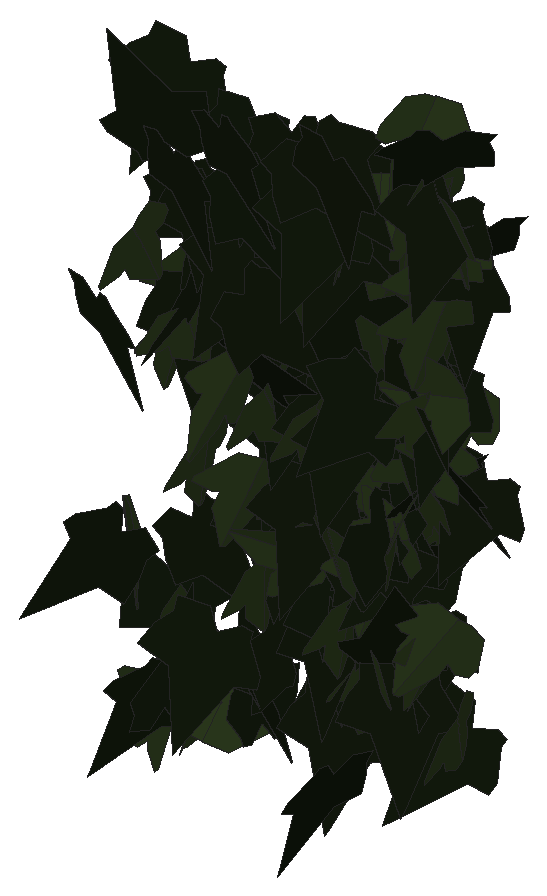
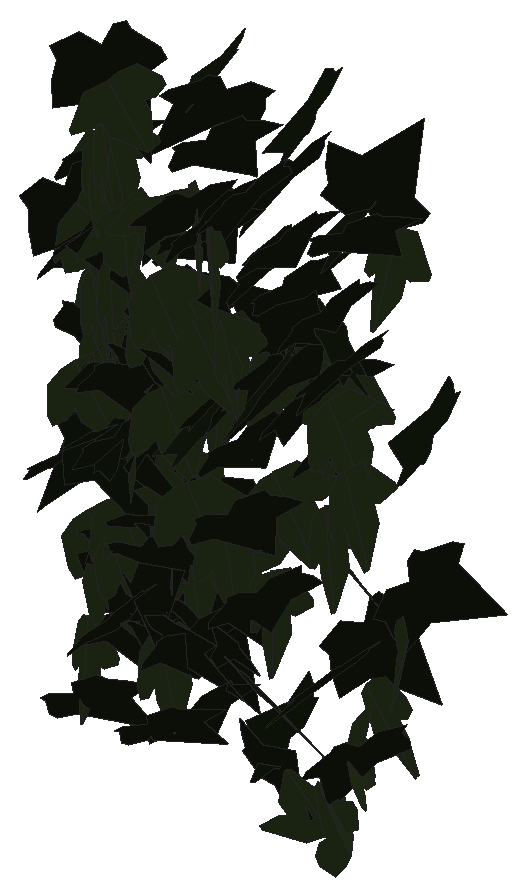
# SketchUp Ruby script. Lengths in inches.
U = 1.inch
M = Sketchup.active_model
def pt(a) = Geom::Point3d.new(a.map { |v| v * U })
def face(e, loops, mat)
  f = e.add_face(loops[0].map { |a| pt(a) })
  loops[1..].each { |l| e.add_face(l.map { |a| pt(a) }).erase! }
  f.material = f.back_material = mat if mat
  f
end
# faces: each face lists its corners as indices into pts; further lists are holes
def faces(e, pts, list, mat = nil) = list.each { |f| face(e, (f[0].is_a?(Array) ? f : [f]).map { |l| l.map { |i| pts[i] } }, mat) }
# xy, xz, yz: faces in a plane at the given z, y or x. An outline is a flat list of corners, or four numbers for a rectangle; further outlines are holes
def ring(l) = l.size == 4 ? [[l[0], l[1]], [l[2], l[1]], [l[2], l[3]], [l[0], l[3]]] : l.each_slice(2).to_a
def flat(e, list, mat, &to3) = list.each { |f| face(e, (f[0].is_a?(Array) ? f : [f]).map { |l| ring(l).map { |u, v| to3.(u, v) } }, mat) }
def xy(e, z, list, mat = nil) = flat(e, list, mat) { |x, y| [x, y, z] }
def xz(e, y, list, mat = nil) = flat(e, list, mat) { |x, z| [x, y, z] }
def yz(e, x, list, mat = nil) = flat(e, list, mat) { |y, z| [x, y, z] }
def lines(e, pts, list) = list.each { |a, b| e.add_line(pt(pts[a]), pt(pts[b])) }
# prism: a flat outline (further loops are holes) pulled along v
def prism(e, loops, v, mat = nil)
  f = face(e, loops, mat); d = Geom::Vector3d.new(v.map { |x| x * U })
  f.pushpull(f.normal.samedirection?(d) ? d.length : -d.length)
end
def box(e, o, s, mat = nil) = prism(e, [[o, [o[0] + s[0], o[1], o[2]], [o[0] + s[0], o[1] + s[1], o[2]], [o[0], o[1] + s[1], o[2]]]], [0, 0, s[2]], mat)
def at(x, y, z, deg = 0) = Geom::Transformation.translation(pt([x, y, z])) * Geom::Transformation.rotation(ORIGIN, Z_AXIS, deg.degrees)
def axes(o, x, y, z) = Geom::Transformation.new([*x, 0, *y, 0, *z, 0, *pt(o).to_a, 1])
def part(name) = M.definitions.add(name)
# library, detail: a bought-in or finely detailed component or shape, given as its bounding box
def library(name, o, s) = part(name).tap { |d| box(d.entities, o, s) }
def detail(e, o, s) = box(e.add_group.entities, o, s)
def put(e, d, t, mat = nil) = e.add_instance(d, t).tap { |i| i.material = mat if mat }
def group(e, t, mat = nil) = e.add_group.tap { |g| g.transformation = t; g.material = mat if mat }.entities
root = M.entities
M.materials.add("efeu1").color = [18, 25, 13]
M.materials.add("efeu2").color = [43, 57, 29]
c1 = part("ivyleaf_9")
p = [[1.54,2.16,1.25],[1.36,2.04,1.19],[-0.21,0.99,0.68],[-0.71,1.11,0.82],[-0.85,0.86,0.67],[-0.8,0.17,0.21],
  [-0.9,-0.01,0.1],[-0.67,-0.16,-0.02],[-0.08,-0.08,-0.05],[-0.03,-0.6,-0.4],[0.65,-0.88,-0.66],[0.83,-0.6,-0.49],
  [1.29,-0.42,-0.43],[1.8125,-0.07,-0.26],[1.21,0.44,0.15]]
faces(c1.entities,p,[[0,1,2,3,4,5,6,7,8,9,10,11,12,13,14]],"efeu1")
c2 = part("ivyleaf_10")
p = [[0,0.5,-0.03],[-0.0625,2.02,-0.43],[-0.19,2.01,-0.46],[-0.54,1.05,-0.29],[-0.52,0.625,-0.18],[-0.83,0.76,-0.28],
  [-1.16,0.64,-0.33],[-1.15,0.33,-0.24],[-0.77,-0.39,0.02],[-0.3,-0.51,0.16],[0.04,-0.48,0.23],[-0.02,2.01,-0.4375],
  [-0.06,2.01,-0.43],[0.04,-0.49,0.23],[0.67,-0.49,0.14],[1.38,0.36,-0.2],[1.375,0.51,-0.24],[0.81,0.65,-0.19],
  [0.62,0.59,-0.15],[0.6,1.09,-0.28],[0.5,1.23,-0.31]]
faces(c2.entities,p,[[0,1,2,3,4,5,6,7,8,9,10],[11,12,0,13,14,15,16,17,18,19,20]],"efeu2")
put(root,c1,axes([18.32,219.18,236.73],[-0.23264,-0.44225,0.01707],[-0.00023,-0.01917,-0.49963],[0.44258,-0.23247,0.00871]))
put(root,c1,axes([16.73,220.26,234.84],[-0.41806,0.26897,-0.05368],[-0.04503,0.02923,0.49711],[0.27055,0.42048,-0.00022]))
put(root,c1,axes([16.32,220.77,234.73],[-0.03728,0.22663,-0.44413],[0.03796,-0.44279,-0.22913],[-0.49716,-0.0508,0.01581]))
put(root,c1,axes([18.61,220.97,234.19],[-0.14053,0.35347,-0.32451],[0.12423,-0.29981,-0.38037],[-0.46348,-0.18754,-0.00356]))
put(root,c2,axes([16.85,221.3,238.65],[-0.03382,-0.35156,0.35392],[0.07856,-0.35406,-0.3442],[0.49263,0.03233,0.07919]))
put(root,c1,axes([15.15,221.35,235.99],[-0.0489,0.0124,-0.49745],[0.08672,-0.49198,-0.02079],[-0.48999,-0.08831,0.04597]))
put(root,c1,axes([16.74,221.28,241.86],[0.30318,-0.39627,0.03242],[0.01873,-0.02649,-0.49895],[0.39716,0.30375,-0.00122]))
put(root,c2,axes([15.68,221.03,240.26],[-0.05258,-0.42552,-0.25722],[0.05175,0.25257,-0.4284],[0.49453,-0.07167,0.01748]))
put(root,c1,axes([18.18,221.54,241.85],[0.10438,-0.44639,0.1996],[0.08744,-0.18377,-0.45671],[0.4811,0.13025,0.0397]))
put(root,c2,axes([15.81,221.17,234.05],[0.30473,-0.15471,-0.36497],[-0.30444,0.2035,-0.34045],[0.25389,0.42971,0.02982]))
put(root,c1,axes([17.23,221.16,239.92],[0.2378,-0.27578,-0.34263],[-0.1,0.3454,-0.34741],[0.42831,0.23376,0.10912]))
put(root,c1,axes([18.04,221.65,241.18],[-0.25106,-0.43024,0.04313],[-0.01388,-0.04182,-0.49805],[0.43218,-0.25128,0.00905]))
put(root,c1,axes([16.83,221.57,238.78],[0.14685,-0.20573,0.4314],[0.35509,-0.25512,-0.24253],[0.31991,0.37761,0.07118]))
put(root,c1,axes([16.91,221.47,241.18],[0.19496,-0.41259,-0.20435],[-0.04645,0.20315,-0.4545],[0.45808,0.1962,0.04089]))
put(root,c1,axes([18.41,221.92,238.65],[-0.21172,-0.34785,0.29012],[-0.08049,-0.28626,-0.40197],[0.44575,-0.21692,0.06522]))
put(root,c1,axes([15.67,221.77,240.95],[0.22727,-0.42698,0.12662],[0.05743,-0.11287,-0.4837],[0.44164,0.2344,-0.00227]))
put(root,c1,axes([16.61,221.98,239.84],[-0.20246,-0.4206,0.17917],[-0.03577,-0.18077,-0.4648],[0.45577,-0.20103,0.04311]))
put(root,c1,axes([15.53,221.71,241.21],[0.2633,0.00372,0.42504],[-0.40216,0.16407,0.24769],[-0.13763,-0.4723,0.08939]))
put(root,c1,axes([17.86,221.6,241.89],[0.0503,-0.31932,-0.38145],[0.12354,0.3794,-0.30132],[0.48188,-0.06394,0.11707]))
put(root,c1,axes([14.42,221.92,238.53],[0.25872,-0.39136,0.17292],[0.09076,-0.14728,-0.46912],[0.41812,0.27413,-0.00517]))
put(root,c2,axes([18.66,222.17,236.97],[-0.07736,-0.11441,-0.48055],[0.13485,-0.47282,0.09087],[-0.47522,-0.11555,0.10402]))
put(root,c2,axes([17.06,221.7,238.32],[-0.07373,-0.42957,-0.24503],[0.04093,0.24158,-0.43585],[0.49284,-0.08433,-0.00046]))
put(root,c2,axes([16.63,222.03,237.02],[-0.23145,-0.40306,0.18432],[-0.07141,-0.17131,-0.46428],[0.43742,-0.24124,0.02174]))
put(root,c1,axes([15.95,221.99,239.49],[-0.39783,0.22915,-0.19804],[0.15833,-0.12137,-0.45848],[-0.25819,-0.4275,0.024]))
put(root,c1,axes([17.97,222.1,238.28],[-0.28766,-0.39412,-0.10918],[0.05279,0.09658,-0.48774],[0.40554,-0.29214,-0.01395]))
put(root,c2,axes([17.95,221.85,236.67],[-0.46075,0.18587,0.05623],[-0.0491,0.02855,-0.49676],[-0.18788,-0.46329,-0.00806]))
put(root,c2,axes([17.62,221.91,238.19],[-0.08403,-0.47039,-0.14723],[0.02547,0.14501,-0.47783],[0.49223,-0.0878,-0.00041]))
put(root,c2,axes([17.97,222.04,235.68],[-0.00171,-0.49775,-0.04733],[-0.00317,0.04734,-0.49774],[0.49999,-0.0014,-0.00332]))
put(root,c1,axes([17.42,222.25,236.87],[-0.39882,-0.26524,-0.1435],[0.11149,0.09139,-0.47877],[0.2802,-0.41388,-0.01375]))
put(root,c2,axes([17.25,222.3,236.01],[-0.22491,-0.02122,-0.44606],[-0.39098,-0.23194,0.20817],[-0.21575,0.44244,0.08774]))
put(root,c1,axes([18.64,222.28,234.76],[-0.12522,-0.47341,-0.10099],[0.03102,0.09625,-0.48967],[0.48307,-0.1289,0.00527]))
put(root,c2,axes([19.17,222.21,239.9],[-0.19706,-0.44281,0.12282],[-0.03389,-0.11927,-0.48438],[0.45828,-0.19923,0.01699]))
put(root,c1,axes([17.65,222.43,240.4],[-0.19809,-0.45502,0.06099],[-0.01773,-0.05879,-0.49622],[0.45875,-0.19875,0.00715]))
put(root,c2,axes([19.22,222.3125,235.72],[-0.33247,-0.21482,0.30548],[-0.19164,-0.25289,-0.38642],[0.32053,-0.37403,0.08582]))
put(root,c2,axes([15.61,222.07,238.72],[-0.21385,-0.42574,-0.15169],[0.06387,0.13767,-0.47641],[0.44742,-0.22314,-0.00449]))
put(root,c1,axes([18.51,222.28,235.16],[0.42159,0.14651,0.22537],[-0.21114,-0.07897,0.4463],[0.16637,-0.47149,-0.00472]))
put(root,c2,axes([14.61,222.26,235.63],[-0.25247,0.37667,-0.21066],[0.07631,-0.20125,-0.4513],[-0.42478,-0.26003,0.04413]))
put(root,c1,axes([19.25,222.17,242.23],[0.03336,0.39852,-0.30011],[-0.14272,-0.28059,-0.38846],[-0.47804,0.11158,0.09503]))
put(root,c2,axes([16.62,222.18,235.7],[0.00602,-0.4867,-0.11438],[0.02004,0.11453,-0.48629],[0.49956,0.00127,0.02088]))
put(root,c1,axes([16.46,222.17,238.91],[0.11594,-0.38414,-0.29831],[-0.02135,0.30236,-0.39765],[0.4859,0.10495,0.05371]))
put(root,c2,axes([18.53,222.24,236.72],[-0.20701,-0.01525,0.45488],[-0.44379,-0.10411,-0.20545],[0.10098,-0.4888,0.02956]))
put(root,c2,axes([19.3,222.2,238.89],[0.1276,0.00772,-0.48338],[-0.46928,0.12209,-0.12193],[0.11615,0.4848,0.03841]))
put(root,c1,axes([19.04,222.56,241.14],[-0.16248,-0.46749,0.0711],[0.00272,-0.07611,-0.49417],[0.47285,-0.1602,0.02727]))
put(root,c1,axes([18.38,222.02,236.96],[0.17794,-0.18481,-0.42916],[-0.16383,0.4054,-0.24251],[0.4376,0.22692,0.08372]))
put(root,c2,axes([17.79,222.23,240.62],[0.26568,-0.39245,-0.15937],[-0.03363,0.16799,-0.46973],[0.42224,0.26032,0.06287]))
put(root,c2,axes([18.22,222.43,236.27],[-0.28434,-0.38052,0.15607],[-0.01846,-0.17774,-0.46698],[0.41086,-0.27132,0.08703]))
put(root,c1,axes([17.55,222.56,233.95],[-0.11709,-0.48526,0.02853],[0.01396,-0.03269,-0.49874],[0.4859,-0.116,0.0212]))
put(root,c1,axes([15.6,222.55,240.0625],[-0.027,-0.49804,0.035],[-0.00041,-0.03503,-0.49877],[0.49927,-0.02696,0.00148]))
put(root,c1,axes([16.13,222.53,234.0625],[0.2143,-0.37408,0.25325],[0.15282,-0.20374,-0.43027],[0.42511,0.26182,0.02701]))
put(root,c2,axes([15.6875,222.29,236.97],[0.01927,-0.48982,-0.09851],[-0.01226,0.09809,-0.49013],[0.49948,0.0213,-0.00823]))
put(root,c1,axes([18.375,222.16,236.11],[-0.46994,0.0383,0.1664],[0.16591,-0.01279,0.4715],[0.04038,0.49837,-0.00069]))
put(root,c2,axes([18.93,222.3,238.61],[-0.168,-0.4604,-0.09903],[0.02599,0.09592,-0.49002],[0.47021,-0.16979,-0.0083]))
put(root,c1,axes([17.86,222.53,239.47],[0.02695,0.18098,-0.46532],[-0.11466,-0.4513,-0.18217],[-0.48593,0.11652,0.01718]))
put(root,c1,axes([16.79,222.51,241.28],[0.08568,-0.48537,-0.08409],[0.00185,0.08567,-0.4926],[0.4926,0.0841,0.01648]))
put(root,c1,axes([17.38,222.57,235.18],[-0.32045,-0.20771,-0.32275],[0.34459,0.02945,-0.36109],[0.16901,-0.45386,0.12427]))
put(root,c2,axes([18.9,222.57,235.4],[0.02016,-0.46392,0.18539],[-0.0018,-0.18561,-0.46427],[0.49959,0.01805,-0.00916]))
put(root,c2,axes([14.94,222.71,234.29],[0.17434,-0.2912,0.36716],[0.22857,-0.28915,-0.33786],[0.4091,0.28565,0.0323]))
put(root,c1,axes([17.29,222.76,240.8],[-0.05143,-0.47217,0.15625],[-0.02724,-0.15417,-0.47486],[0.4966,-0.05736,-0.00986]))
put(root,c1,axes([15.25,222.66,238.54],[0.00132,-0.49997,-0.00532],[0.00004,0.00532,-0.49997],[0.5,0.00132,0.00006]))
put(root,c1,axes([16.8,222.4,234.52],[-0.38182,0.27662,0.16641],[-0.16391,0.05592,-0.46905],[-0.27811,-0.41274,0.04798]))
put(root,c1,axes([19.02,222.61,238.79],[-0.40371,-0.20599,-0.21116],[0.17929,0.11287,-0.4529],[0.23425,-0.44139,-0.01727]))
put(root,c2,axes([18.41,222.1875,234.71],[-0.1228,0.23164,-0.42575],[-0.21963,0.36493,0.2619],[0.43207,0.25134,0.01212]))
put(root,c1,axes([18.54,222.65,239.01],[0.17897,-0.46572,0.03273],[0.00764,-0.03213,-0.49891],[0.46681,0.17908,-0.00439]))
put(root,c1,axes([15.02,222.8,241.48],[-0.29136,-0.40062,0.06792],[0.01585,-0.09471,-0.49069],[0.40603,-0.28378,0.06789]))
put(root,c1,axes([17.0625,222.49,238.44],[0.15996,-0.4199,-0.21932],[-0.02937,0.22225,-0.44693],[0.47281,0.15586,0.04644]))
put(root,c1,axes([16.66,222.79,238.05],[-0.11535,-0.48244,0.06282],[-0.00827,-0.0626,-0.496],[0.48644,-0.11547,0.00646]))
put(root,c2,axes([18.73,222.45,237.8],[-0.42978,-0.21282,-0.14142],[0.13678,0.04214,-0.47908],[0.21583,-0.45048,0.022]))
put(root,c2,axes([18.22,222.45,239.13],[-0.49878,0.0219,0.0272],[-0.02717,0.00119,-0.49926],[-0.02193,-0.49952,0]))
put(root,c1,axes([16.02,222.83,241.01],[-0.06861,-0.49096,0.0652],[0.01069,-0.06728,-0.49534],[0.49516,-0.06657,0.01973]))
put(root,c2,axes([18.9,222.68,240.15],[-0.25963,-0.40554,0.13465],[-0.02665,-0.14188,-0.47871],[0.42647,-0.25575,0.05206]))
put(root,c1,axes([18.48,222.9375,236.29],[-0.39007,-0.2742,0.15052],[-0.04933,-0.18366,-0.46242],[0.30889,-0.37561,0.11623]))
put(root,c2,axes([18.74,222.47,237.33],[-0.41504,0.14577,0.23768],[-0.22998,0.06199,-0.43962],[-0.15764,-0.47424,0.01559]))
put(root,c2,axes([17.92,222.67,234.65],[-0.05427,-0.49609,0.0309],[-0.00255,-0.03081,-0.49904],[0.49704,-0.05432,0.00081]))
put(root,c2,axes([18.625,222.71,242.1],[0.24829,0.38345,-0.20326],[-0.16623,-0.13229,-0.45262],[-0.4009,0.29234,0.06179]))
put(root,c2,axes([17.4,222.76,236.92],[-0.35589,-0.29795,0.18592],[-0.0752,-0.19391,-0.45469],[0.34306,-0.3516,0.09321]))
put(root,c2,axes([18.71,222.73,241.32],[-0.07956,-0.48753,0.07734],[-0.00182,-0.07805,-0.49387],[0.49363,-0.07886,0.01064]))
put(root,c1,axes([18.23,222.5,236.19],[0.16253,0.43439,-0.18679],[-0.06704,-0.17435,-0.4638],[-0.46807,0.17581,0.00157]))
put(root,c1,axes([18.03,222.9,236.13],[-0.3381,-0.35851,-0.08458],[0.07662,0.04385,-0.49215],[0.3603,-0.34575,0.02528]))
put(root,c2,axes([15.27,222.6,232.95],[0.21321,-0.42925,0.14244],[-0.06441,0.12705,0.47928],[-0.44765,-0.22273,-0.00111]))
put(root,c2,axes([16.91,222.74,236.62],[-0.14033,-0.47918,0.02631],[0.00625,-0.02924,-0.49911],[0.47986,-0.13975,0.01419]))
put(root,c2,axes([19.15,222.55,234.36],[0.05969,-0.4314,-0.24562],[-0.02822,0.24404,-0.43549],[0.49562,0.06585,0.00478]))
put(root,c2,axes([19,222.6,241.03],[-0.40372,0.29431,0.01987],[-0.01497,0.0132,-0.4996],[-0.2946,-0.40399,-0.00185]))
put(root,c1,axes([18.48,222.89,238.49],[-0.16875,-0.46052,-0.0972],[0.04425,0.08728,-0.49033],[0.46858,-0.17409,0.0113]))
put(root,c2,axes([17.74,222.83,238.14],[-0.29924,-0.36542,0.16409],[-0.02938,-0.18424,-0.46389],[0.39949,-0.28727,0.08879]))
put(root,c2,axes([16.86,222.7,239.33],[0.07444,-0.48921,-0.07162],[-0.01151,0.07069,-0.49484],[0.49429,0.07532,-0.00074]))
put(root,c1,axes([17.34,222.92,235.21],[-0.09479,-0.48967,-0.03521],[0.00683,0.03454,-0.49876],[0.49089,-0.09504,0.00014]))
put(root,c2,axes([18.35,222.92,236.05],[-0.1158,-0.42744,0.23213],[-0.00213,-0.23816,-0.43963],[0.4864,-0.10281,0.05334]))
put(root,c1,axes([18.85,222.68,237.4],[-0.12179,0.43645,-0.21137],[-0.00194,-0.21837,-0.44979],[-0.48494,-0.10874,0.05489]))
put(root,c1,axes([17.47,222.76,241.05],[0.04307,-0.43487,-0.24297],[0.05003,0.24642,-0.43217],[0.49562,0.01292,0.06474]))
put(root,c2,axes([17.88,222.75,240.79],[0.29582,0.39976,-0.05175],[-0.02855,-0.04325,-0.49731],[-0.40209,0.29718,-0.00276]))
put(root,c1,axes([18.37,223.02,237.6],[-0.13153,-0.48114,0.03467],[-0.01039,-0.0331,-0.49879],[0.48228,-0.13194,-0.00129]))
put(root,c2,axes([18.37,222.82,236.43],[-0.23736,-0.42931,0.09672],[-0.05102,-0.0823,-0.49053],[0.4371,-0.24274,-0.00473]))
put(root,c2,axes([15.1,222.88,238.9],[-0.11733,-0.4659,0.13846],[-0.03044,-0.13511,-0.48044],[0.48508,-0.12117,0.00334]))
put(root,c2,axes([18.71,222.76,241.42],[0.10212,-0.48614,-0.05695],[0.00366,0.05893,-0.4965],[0.48945,0.10099,0.01559]))
put(root,c1,axes([18.95,222.99,240.14],[0.02148,-0.4975,0.04507],[-0.00138,-0.04517,-0.49795],[0.49954,0.02127,-0.00331]))
put(root,c2,axes([18.66,222.93,240.97],[0.12768,-0.45316,0.16835],[0.09196,-0.14818,-0.4686],[0.4746,0.15063,0.0455]))
put(root,c1,axes([17.83,222.93,235.09],[-0.49264,-0.07428,0.04229],[-0.04224,-0.00353,-0.4982],[0.07432,-0.49444,-0.0028]))
put(root,c2,axes([18.92,222.97,240.52],[0.06608,0.37175,-0.32777],[-0.10932,-0.3116,-0.37544],[-0.48341,0.12128,0.0401]))
put(root,c2,axes([18.81,222.82,239.39],[0.06332,-0.49571,-0.01625],[0.00375,0.01686,-0.4997],[0.49596,0.06317,0.00585]))
put(root,c1,axes([16.23,222.97,236.18],[-0.10067,-0.48312,-0.08039],[0.01245,0.07952,-0.49348],[0.4896,-0.10136,-0.00398]))
put(root,c2,axes([17.77,222.95,239.72],[-0.14414,-0.44623,0.17351],[-0.0177,-0.17612,-0.46762],[0.47845,-0.14094,0.03497]))
put(root,c1,axes([16.15,223.03,238.96],[0.15914,-0.45611,0.129],[0.04762,-0.12,-0.48304],[0.4716,0.16603,0.00525]))
put(root,c1,axes([17.72,223.15,233.95],[-0.35424,-0.33234,0.1186],[-0.03191,-0.13719,-0.47975],[0.35142,-0.34746,0.07599]))
put(root,c1,axes([15.49,222.96,239.15],[0.09286,-0.4866,-0.06782],[-0.00256,0.06854,-0.49527],[0.49129,0.09233,0.01024]))
put(root,c1,axes([18.87,223.13,233.95],[-0.38902,-0.29839,0.09813],[-0.05804,-0.08524,-0.48925],[0.3087,-0.39204,0.03169]))
put(root,c1,axes([16.25,222.62,233.43],[0.16316,0.07036,0.46736],[-0.27922,0.41327,0.03526],[-0.38133,-0.2725,0.17415]))
put(root,c2,axes([15.51,222.65,233.13],[0.42539,0.18134,-0.19014],[0.13988,0.15,0.456],[0.22243,-0.44115,0.07689]))
put(root,c1,axes([16.54,223.11,237.22],[-0.25188,-0.43161,0.01631],[-0.00696,-0.01482,-0.49973],[0.43187,-0.25197,0.00146]))
put(root,c1,axes([18.77,222.72,237.56],[0.48886,-0.04402,-0.0953],[-0.09594,-0.00316,-0.4907],[0.0426,0.49805,-0.01154]))
put(root,c1,axes([19.05,223.21,237.22],[-0.19153,-0.43487,0.15558],[0.02884,-0.17935,-0.46583],[0.46096,-0.16947,0.09378]))
put(root,c2,axes([17.77,222.97,239.4],[-0.15648,-0.46305,0.10536],[-0.01335,-0.1066,-0.48832],[0.47469,-0.15564,0.02099]))
put(root,c2,axes([14.83,222.94,238.05],[-0.00933,-0.49884,0.03278],[-0.00589,-0.03267,-0.4989],[0.49988,-0.00969,-0.00526]))
put(root,c2,axes([18.84,223.08,238.26],[-0.29723,-0.33374,0.22422],[-0.01112,-0.27191,-0.41946],[0.40191,-0.25433,0.15422]))
put(root,c1,axes([14.7,222.96,234.59],[0.00431,-0.45931,-0.19752],[0.03363,0.19735,-0.45817],[0.49885,-0.00934,0.0326]))
put(root,c1,axes([14.93,222.94,239.8125],[0.15555,-0.45226,-0.14583],[0.02542,0.16115,-0.47264],[0.47451,0.13962,0.07312]))
put(root,c1,axes([15.1,222.85,235.49],[0.24636,-0.38906,-0.19478],[0.0268,0.23699,-0.43945],[0.43427,0.20609,0.13763]))
put(root,c1,axes([16.97,222.98,238.35],[0.29704,-0.40177,0.01859],[0.04425,0.00968,-0.49794],[0.39976,0.29747,0.04131]))
put(root,c1,axes([19.18,222.9375,240.65],[-0.11463,0.38529,-0.29735],[-0.02064,-0.30906,-0.3925],[-0.48625,-0.07771,0.08676]))
put(root,c1,axes([18.34,223.21,235.18],[-0.05371,-0.47965,0.13057],[0.03577,-0.13472,-0.48018],[0.49582,-0.04224,0.04879]))
put(root,c2,axes([18.375,222.92,240.57],[0.0722,0.48424,-0.1015],[-0.05551,-0.094,-0.48794],[-0.49164,0.08172,0.04018]))
put(root,c1,axes([17.92,223.14,238.92],[-0.45587,-0.18363,-0.09202],[0.11018,-0.02959,-0.48681],[0.17334,-0.46412,0.06744]))
put(root,c2,axes([18.51,222.91,239.67],[0.09266,-0.48617,-0.07108],[0.0285,0.07753,-0.49313],[0.49051,0.08734,0.04208]))
put(root,c2,axes([17.05,222.84,240.64],[0.21482,-0.41113,-0.18662],[-0.03977,0.18863,-0.46134],[0.44974,0.21306,0.04835]))
put(root,c2,axes([16.99,223.08,239.42],[-0.15457,-0.44077,0.17841],[-0.04234,-0.17409,-0.4668],[0.47362,-0.15941,0.01649]))
put(root,c1,axes([18.09,223.13,238.72],[-0.17837,-0.45487,-0.10619],[0.05782,0.09129,-0.48818],[0.46351,-0.18644,0.02003]))
